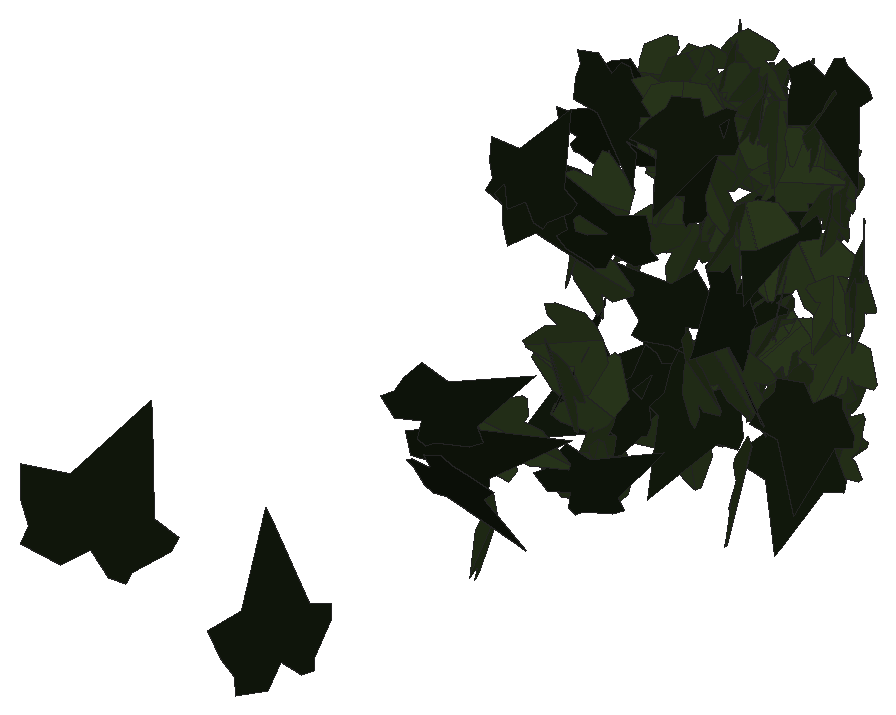
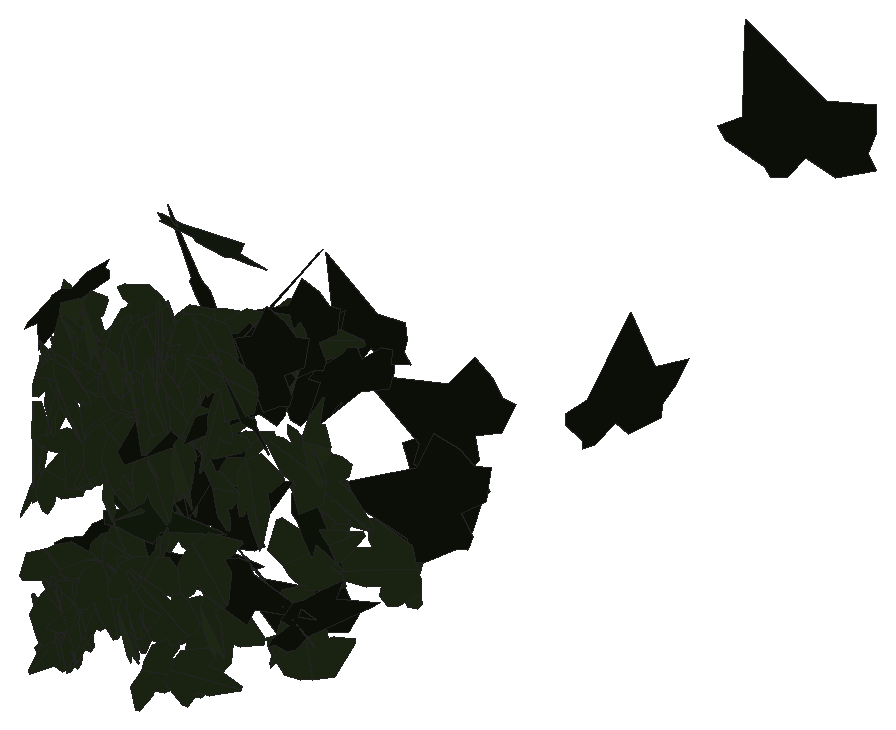
# SketchUp Ruby script. Lengths in inches.
U = 1.inch
M = Sketchup.active_model
def pt(a) = Geom::Point3d.new(a.map { |v| v * U })
def face(e, loops, mat)
  f = e.add_face(loops[0].map { |a| pt(a) })
  loops[1..].each { |l| e.add_face(l.map { |a| pt(a) }).erase! }
  f.material = f.back_material = mat if mat
  f
end
# faces: each face lists its corners as indices into pts; further lists are holes
def faces(e, pts, list, mat = nil) = list.each { |f| face(e, (f[0].is_a?(Array) ? f : [f]).map { |l| l.map { |i| pts[i] } }, mat) }
# xy, xz, yz: faces in a plane at the given z, y or x. An outline is a flat list of corners, or four numbers for a rectangle; further outlines are holes
def ring(l) = l.size == 4 ? [[l[0], l[1]], [l[2], l[1]], [l[2], l[3]], [l[0], l[3]]] : l.each_slice(2).to_a
def flat(e, list, mat, &to3) = list.each { |f| face(e, (f[0].is_a?(Array) ? f : [f]).map { |l| ring(l).map { |u, v| to3.(u, v) } }, mat) }
def xy(e, z, list, mat = nil) = flat(e, list, mat) { |x, y| [x, y, z] }
def xz(e, y, list, mat = nil) = flat(e, list, mat) { |x, z| [x, y, z] }
def yz(e, x, list, mat = nil) = flat(e, list, mat) { |y, z| [x, y, z] }
def lines(e, pts, list) = list.each { |a, b| e.add_line(pt(pts[a]), pt(pts[b])) }
# prism: a flat outline (further loops are holes) pulled along v
def prism(e, loops, v, mat = nil)
  f = face(e, loops, mat); d = Geom::Vector3d.new(v.map { |x| x * U })
  f.pushpull(f.normal.samedirection?(d) ? d.length : -d.length)
end
def box(e, o, s, mat = nil) = prism(e, [[o, [o[0] + s[0], o[1], o[2]], [o[0] + s[0], o[1] + s[1], o[2]], [o[0], o[1] + s[1], o[2]]]], [0, 0, s[2]], mat)
def at(x, y, z, deg = 0) = Geom::Transformation.translation(pt([x, y, z])) * Geom::Transformation.rotation(ORIGIN, Z_AXIS, deg.degrees)
def axes(o, x, y, z) = Geom::Transformation.new([*x, 0, *y, 0, *z, 0, *pt(o).to_a, 1])
def part(name) = M.definitions.add(name)
# library, detail: a bought-in or finely detailed component or shape, given as its bounding box
def library(name, o, s) = part(name).tap { |d| box(d.entities, o, s) }
def detail(e, o, s) = box(e.add_group.entities, o, s)
def put(e, d, t, mat = nil) = e.add_instance(d, t).tap { |i| i.material = mat if mat }
def group(e, t, mat = nil) = e.add_group.tap { |g| g.transformation = t; g.material = mat if mat }.entities
root = M.entities
M.materials.add("efeu1").color = [18, 25, 13]
M.materials.add("efeu2").color = [43, 57, 29]
c1 = part("ivyleaf_9")
p = [[1.54,2.16,1.25],[1.36,2.04,1.19],[-0.21,0.99,0.68],[-0.71,1.11,0.82],[-0.85,0.86,0.67],[-0.8,0.17,0.21],
  [-0.9,-0.01,0.1],[-0.67,-0.16,-0.02],[-0.08,-0.08,-0.05],[-0.03,-0.6,-0.4],[0.65,-0.88,-0.66],[0.83,-0.6,-0.49],
  [1.29,-0.42,-0.43],[1.8125,-0.07,-0.26],[1.21,0.44,0.15]]
faces(c1.entities,p,[[0,1,2,3,4,5,6,7,8,9,10,11,12,13,14]],"efeu1")
c2 = part("ivyleaf_10")
p = [[0,0.5,-0.03],[-0.0625,2.02,-0.43],[-0.19,2.01,-0.46],[-0.54,1.05,-0.29],[-0.52,0.625,-0.18],[-0.83,0.76,-0.28],
  [-1.16,0.64,-0.33],[-1.15,0.33,-0.24],[-0.77,-0.39,0.02],[-0.3,-0.51,0.16],[0.04,-0.48,0.23],[-0.02,2.01,-0.4375],
  [-0.06,2.01,-0.43],[0.04,-0.49,0.23],[0.67,-0.49,0.14],[1.38,0.36,-0.2],[1.375,0.51,-0.24],[0.81,0.65,-0.19],
  [0.62,0.59,-0.15],[0.6,1.09,-0.28],[0.5,1.23,-0.31]]
faces(c2.entities,p,[[0,1,2,3,4,5,6,7,8,9,10],[11,12,0,13,14,15,16,17,18,19,20]],"efeu2")
put(root,c1,axes([508.35,118,168.35],[-0.80992,-0.06692,0.86891],[0.90068,-0.17166,0.7642],[0.0905,1.10948,0.17065]))
put(root,c1,axes([509.34,122.875,163.92],[-0.48865,-0.70509,0.59701],[0.48935,0.38106,0.85817],[-0.85134,0.62373,0.1506]))
put(root,c1,axes([508.68,128.82,165.375],[0.90393,0.02313,0.05304],[0.05509,0.00026,-0.87078],[-0.02495,0.83852,-0.00119]))
put(root,c1,axes([508.39,128.84,166.52],[0.12124,-0.07324,0.85207],[0.88337,0.09754,-0.10749],[-0.09411,0.82118,0.08876]))
put(root,c2,axes([508.98,130.13,163.63],[0.02278,-0.05399,0.83347],[0.51986,-0.64094,-0.05808],[0.69446,0.48156,0.01614]))
put(root,c1,axes([508.17,129.62,165.1],[0.35904,0.07136,0.84573],[0.85849,0.17155,-0.35361],[-0.20067,0.86162,0.00036]))
put(root,c2,axes([507.93,131.74,164.78],[0.18066,0.06133,0.76871],[0.69913,0.35775,-0.18324],[-0.39096,0.66808,0.02755]))
put(root,c1,axes([508.29,132.27,170.14],[-0.51612,0.1888,0.56428],[0.50132,-0.28891,0.52976],[0.36555,0.66279,0.07018]))
put(root,c2,axes([508.98,132.43,166.39],[-0.65347,0.4003,-0.0382],[0.03066,-0.02366,-0.7545],[-0.43305,-0.60571,0.00423]))
put(root,c2,axes([509.32,132.85,166.89],[0.3552,-0.01331,-0.7252],[-0.73009,0.18356,-0.33524],[0.18529,0.74881,0.06929]))
put(root,c1,axes([509.14,132.74,163.37],[0.06641,-0.08518,0.72361],[0.75558,0.05107,-0.0578],[-0.04727,0.69662,0.09272]))
put(root,c2,axes([509.73,133.18,170.08],[0.14189,0.10505,0.76899],[-0.6514,-0.42782,0.17466],[0.47566,-0.61722,0.00981]))
put(root,c1,axes([508.04,132.89,170.07],[0.10578,-0.46737,-0.57412],[-0.04606,0.55237,-0.49423],[0.77981,0.09603,0.04869]))
put(root,c1,axes([509.67,133.29,168.9375],[0.44786,-0.10823,0.64797],[-0.64789,0.16839,0.44567],[-0.21608,-0.72924,0.00674]))
put(root,c2,axes([511.58,133.45,166.6875],[-0.04078,-0.01524,0.83192],[0.79397,-0.24982,0.03434],[0.24885,0.79457,0.02675]))
put(root,c2,axes([509.28,133.35,165.19],[0.39765,0.27834,0.62435],[-0.52526,-0.35203,0.47995],[0.4846,-0.60995,0.0079]))
put(root,c2,axes([508.94,133.43,163.01],[-0.62821,-0.33296,0.11741],[0.11317,0.04415,0.69689],[-0.36245,0.59088,0.01409]))
put(root,c1,axes([509.01,133.58,166.8],[-0.47671,0.28129,-0.44047],[0.36622,-0.25504,-0.5437],[-0.40915,-0.55602,0.02655]))
put(root,c1,axes([511.47,133.99,172.29],[-0.67868,-0.45976,-0.28208],[0.50624,-0.2748,-0.64498],[0.27585,-0.62685,0.48964]))
put(root,c2,axes([508.27,134.18,168.65],[0.18556,-0.29901,0.60908],[0.34703,-0.48995,-0.35818],[0.61961,0.36395,0.01821]))
put(root,c2,axes([509.19,133.26,164.01],[-0.00215,0.29168,0.64976],[-0.21374,0.59824,-0.29112],[-0.71332,-0.18014,0.08528]))
put(root,c2,axes([512.32,134.26,164.41],[0.34093,-0.41324,0.65956],[0.42905,-0.501,-0.53567],[0.64939,0.54796,0.00764]))
put(root,c2,axes([508.41,134.07,167.86],[0.00518,-0.01966,-0.8024],[0.7144,-0.39739,0.01481],[-0.42943,-0.66135,0.01495]))
put(root,c1,axes([511.13,133.92,170.55],[-0.23168,0.46867,0.64282],[0.27772,-0.57975,0.52278],[0.74548,0.36163,0.00502]))
put(root,c1,axes([508.42,133.89,170.88],[0.41242,-0.12481,0.56756],[0.55698,-0.17856,-0.41778],[0.23521,0.64169,-0.00586]))
put(root,c1,axes([508.36,134.66,164.6],[-0.35515,-0.43073,0.55439],[-0.32213,-0.45204,-0.55758],[0.62378,-0.47868,0.0277]))
put(root,c1,axes([508.78,134.43,172.15],[0.22842,-0.79499,0.10746],[0.0454,-0.09874,-0.827],[0.80094,0.23232,0.01623]))
put(root,c1,axes([511.7,134.77,167.94],[0.24173,-0.33736,-0.74303],[0.53299,-0.52154,0.41019],[-0.61792,-0.58183,0.06315]))
put(root,c1,axes([510.03,133.97,165.125],[-0.53393,0.49004,0.36474],[-0.27345,0.24144,-0.72469],[-0.54626,-0.59985,0.00627]))
put(root,c1,axes([510.9375,134.84,165.33],[-0.6752,-0.49233,-0.06076],[0.04867,0.03638,-0.83563],[0.49367,-0.67695,-0.00072]))
put(root,c1,axes([511.62,135.08,165.79],[0.17181,-0.35272,0.70217],[0.29434,-0.63754,-0.39228],[0.72858,0.34074,-0.00711]))
put(root,c2,axes([511.5,135.17,169.18],[-0.00977,0.06863,-0.73588],[0.02267,-0.73557,-0.0689],[-0.73873,-0.02348,0.00762]))
put(root,c2,axes([508.27,134.61,170.98],[-0.45655,0.59002,-0.14212],[0.07712,-0.11693,-0.75479],[-0.64953,-0.4286,0.01028]))
put(root,c2,axes([509.99,134.88,170.45],[0.67734,-0.34388,-0.02023],[-0.01714,0.01152,-0.74386],[0.37159,0.62736,0.00257]))
put(root,c2,axes([511.49,134.71,166.34],[-0.77683,0.00632,-0.33487],[0.33492,0.01008,-0.77676],[-0.00182,-0.84587,-0.01176]))
put(root,c1,axes([509.87,135.07,165.32],[-0.22912,-0.18393,-0.64949],[-0.54361,-0.37024,0.29123],[-0.44593,0.54584,-0.02132]))
put(root,c1,axes([510.06,135.12,166.57],[0.08917,-0.00641,0.70103],[-0.72077,0.09487,0.08595],[-0.10254,-0.67245,0.00544]))
put(root,c2,axes([508.96,134.93,171.56],[0.40955,0.49453,0.15605],[0.09784,0.11962,-0.64811],[-0.54949,0.38989,0.00091]))
put(root,c2,axes([510.25,135.03,164.26],[-0.66233,-0.4927,-0.06058],[0.04817,0.03673,-0.82549],[0.49407,-0.66408,-0.00072]))
put(root,c2,axes([510.58,135.2,170.14],[0.55853,-0.06915,0.5227],[0.54787,0.06062,-0.53419],[0.00753,0.7186,0.09536]))
put(root,c2,axes([511.61,135.47,169.33],[-0.72881,-0.23556,-0.29548],[0.39752,-0.38621,-0.5762],[0.02918,-0.62205,0.46963]))
put(root,c2,axes([509.49,135.64,168.47],[0.03444,0.17741,0.60964],[-0.1004,-0.57878,0.18744],[0.65378,-0.09822,-0.00333]))
put(root,c1,axes([513.06,135.61,165.42],[-0.22405,-0.73146,-0.03867],[0.01161,0.03689,-0.76501],[0.73239,-0.22435,0.00029]))
put(root,c1,axes([512.8125,135.66,164.3125],[-0.38444,-0.65055,-0.08061],[0.03708,0.07173,-0.75564],[0.65448,-0.3862,-0.00455]))
put(root,c2,axes([509.78,135.42,171.54],[0.70654,0.34748,0.00337],[0.00302,0.00164,-0.77039],[-0.37529,0.65421,0.00014]))
put(root,c2,axes([508.79,135.49,168.23],[0.09695,-0.71984,-0.06707],[-0.01625,0.06549,-0.7263],[0.72277,0.09803,-0.00733]))
put(root,c1,axes([511.91,136.09,169.36],[-0.60215,-0.49793,-0.32111],[0.58361,-0.27233,-0.55807],[0.24451,-0.57621,0.54124]))
put(root,c1,axes([507.98,135.58,171],[0.39146,-0.08579,0.64541],[0.63165,-0.13259,-0.40074],[0.15789,0.74311,0.00301]))
put(root,c2,axes([512.17,135.875,165.51],[-0.12287,-0.7097,-0.14698],[0.03958,0.14228,-0.72011],[0.72368,-0.12828,0.01443]))
put(root,c2,axes([510.89,136.42,168.84],[0.06532,-0.5106,0.52642],[0.10378,-0.51675,-0.5141],[0.72599,0.11981,0.02613]))
put(root,c1,axes([508.44,135.55,170.95],[0.58265,0.44586,0.21678],[0.16744,0.13789,-0.73363],[-0.46664,0.60619,0.00743]))
put(root,c2,axes([510.58,136.33,168.28],[0.18518,-0.45942,-0.41947],[0.22483,-0.34999,0.50664],[-0.6208,-0.26379,0.05836]))
put(root,c1,axes([511.39,136.38,166.97],[-0.69309,0.24528,-0.00723],[-0.18122,-0.45286,-0.50823],[-0.19336,-0.45476,0.50222]))
put(root,c2,axes([511.875,136.22,168.48],[0.07784,-0.63698,0.05729],[0.01392,-0.05602,-0.64168],[0.6394,0.07876,0.00699]))
put(root,c2,axes([509.89,136.4,168.78],[0.39324,-0.22962,0.57025],[0.5117,-0.2529,-0.4547],[0.34069,0.64488,0.02473]))
put(root,c1,axes([509.76,135.77,169.42],[0.23918,0.65563,-0.02342],[-0.01099,-0.02034,-0.7197],[-0.70841,0.22168,0.00325]))
put(root,c2,axes([509.66,136.08,170.94],[-0.65568,-0.31948,-0.21323],[0.19931,0.07762,-0.72917],[0.32834,-0.68509,0.01682]))
put(root,c2,axes([510.75,136.34,170.75],[-0.59006,-0.45413,0.18457],[-0.12783,-0.1363,-0.74402],[0.47325,-0.60305,0.02917]))
put(root,c2,axes([509.09,136.52,169.55],[0.16551,0.40545,0.51264],[-0.24613,-0.43875,0.44902],[0.64387,-0.27195,0.03987]))
put(root,c2,axes([509.13,136.52,171.45],[-0.17803,0.04055,-0.73109],[0.60563,-0.4147,-0.17048],[-0.41151,-0.62786,0.06538]))
put(root,c2,axes([511.92,136.32,170.02],[0.14883,-0.18809,-0.62528],[0.63899,-0.08999,0.17916],[-0.13434,-0.63642,0.15947]))
put(root,c2,axes([511.13,136.3125,171.5625],[0.18509,-0.59652,-0.18005],[-0.01518,0.18345,-0.6234],[0.62292,0.18172,0.03831]))
put(root,c2,axes([512.89,136.8125,167.43],[-0.17313,-0.38144,0.48849],[0.14492,-0.51805,-0.35316],[0.60259,0.015,0.22528]))
put(root,c2,axes([511.49,136.53,171.25],[0.01761,0.63966,-0.25407],[-0.00226,-0.2541,-0.63989],[-0.68827,0.0172,-0.0044]))
put(root,c2,axes([512.28,136.96,171.24],[-0.06052,-0.22027,-0.66498],[0.0953,-0.66384,0.21122],[-0.694,-0.07195,0.087]))
put(root,c1,axes([508.8,136.01,170.53],[-0.56172,0.25617,-0.54675],[-0.5119,0.19396,0.61679],[0.32019,0.7595,0.0269]))
put(root,c2,axes([512.14,136.64,168.18],[-0.69831,-0.24088,-0.42554],[0.5121,-0.29156,-0.60075],[0.02672,-0.70745,0.39248]))
put(root,c2,axes([509.33,136.41,171.875],[-0.45719,-0.34432,-0.23724],[0.19586,0.13853,-0.56746],[0.40077,-0.46049,0.00668]))
put(root,c2,axes([511.15,136.97,166.46],[0.0697,-0.43926,0.49745],[0.10397,-0.48679,-0.44441],[0.65544,0.12392,0.0176]))
put(root,c2,axes([512.68,136.96,169.6],[-0.06758,0.31516,-0.62508],[0.09975,-0.61725,-0.32199],[-0.6929,-0.11959,0.01461]))
put(root,c2,axes([508.88,136.8125,165.52],[0.27343,-0.45159,0.26163],[0.13523,-0.21821,-0.53842],[0.54167,0.28243,0.00235]))
put(root,c2,axes([511.52,136.93,169.79],[-0.24651,-0.50319,0.3595],[0.02692,-0.39538,-0.53494],[0.61783,-0.18355,0.16675]))
put(root,c2,axes([510.37,136.78,168.53],[-0.05221,-0.63909,0.12976],[-0.00411,-0.12985,-0.64119],[0.65212,-0.05199,0.00635]))
put(root,c2,axes([508.14,136.67,171.09],[0.10248,-0.06125,-0.70118],[0.68978,-0.13223,0.11236],[-0.14003,-0.69618,0.04035]))
put(root,c2,axes([510.24,136.76,166.54],[-0.08078,0.57633,-0.22736],[0.01515,-0.21857,-0.60425],[-0.66554,-0.07492,0.01384]))
put(root,c2,axes([509.71,136.95,170.48],[-0.25952,-0.53289,0.29073],[-0.0605,-0.2919,-0.58905],[0.60402,-0.2582,0.06591]))
put(root,c2,axes([511.76,136.9,165.31],[-0.066,0.58529,-0.36019],[0.04057,-0.3579,-0.589],[-0.68605,-0.07747,-0.00018]))
put(root,c2,axes([512.9,136.68,169.95],[-0.12207,-0.67095,-0.14265],[0.03341,0.1389,-0.68192],[0.68513,-0.12632,0.00783]))
put(root,c2,axes([510.39,136.93,171.68],[-0.30879,-0.54295,0.15479],[0.03751,-0.19577,-0.61186],[0.56334,-0.28458,0.12559]))
put(root,c2,axes([510.83,137.04,171.22],[0.00059,-0.57979,0.27924],[0.03094,-0.27889,-0.57913],[0.64279,0.01396,0.02762]))
put(root,c2,axes([509.48,136.94,169.08],[0.22232,-0.61813,0.11505],[0.05183,-0.1036,-0.65676],[0.62661,0.22788,0.01351]))
put(root,c2,axes([511.36,137.05,165.83],[-0.59465,0.23653,0.29391],[-0.39189,-0.43671,-0.35511],[0.06953,-0.43854,0.51216]))
put(root,c2,axes([510.58,137,171.65],[0.06509,-0.62126,0.15416],[0.05715,-0.1487,-0.62337],[0.63755,0.07676,0.04014]))
put(root,c2,axes([510.86,136.92,170.93],[-0.41578,0.25289,-0.44889],[0.38793,-0.22596,-0.4866],[-0.33907,-0.56861,-0.00627]))
put(root,c2,axes([511.21,136.64,170.25],[0.28524,0.60614,-0.14799],[0.02386,0.152,0.66858],[0.62349,-0.28312,0.04212]))
put(root,c2,axes([510.24,136.875,172.23],[-0.451,0.06488,-0.51754],[0.50231,-0.13028,-0.45406],[-0.14051,-0.674,0.03795]))
put(root,c2,axes([511.18,137.12,167.42],[0.42631,-0.41907,0.26503],[0.17459,-0.20028,-0.5975],[0.46409,0.4603,-0.01868]))
put(root,c2,axes([513.08,137.11,167.57],[-0.12451,0.50445,-0.38803],[0.0724,-0.38159,-0.51931],[-0.63229,-0.14303,0.01694]))
put(root,c1,axes([509.75,136.57,169.98],[0.02466,-0.13874,-0.68701],[0.05892,0.65919,-0.14202],[0.72662,-0.04874,0.03483]))
put(root,c2,axes([511.36,137.09,165.79],[-0.5098,-0.36935,-0.29326],[0.4735,-0.22076,-0.46254],[0.16633,-0.50358,0.41786]))
put(root,c1,axes([512.23,137.1,172.13],[0.17291,-0.73216,-0.23493],[-0.03547,0.23295,-0.75208],[0.76811,0.17557,0.01816]))
put(root,c2,axes([508.73,137.24,167.16],[-0.17583,-0.55983,0.28973],[-0.01528,-0.29692,-0.58299],[0.63017,-0.1634,0.0667]))
put(root,c2,axes([510.04,136.89,170.49],[-0.41989,-0.51086,-0.1733],[0.10947,0.13435,-0.66128],[0.52823,-0.43393,-0.00072]))
put(root,c2,axes([509.6875,137.17,171.06],[0.46251,-0.12014,0.4827],[0.46412,-0.13288,-0.47779],[0.17895,0.65517,-0.00839]))
put(root,c2,axes([512.4375,137.12,163.58],[0.46779,-0.20882,-0.40512],[0.36829,-0.16879,0.51227],[-0.26849,-0.59536,-0.00314]))
put(root,c2,axes([511.6,137.17,170.59],[-0.01252,-0.01891,0.72738],[0.72515,-0.0603,0.01092],[0.05998,0.72499,0.01988]))
put(root,c2,axes([508.66,136.84,168.59],[0.33387,-0.06081,0.61841],[-0.5927,0.17971,0.33766],[-0.18665,-0.67942,0.03396]))
put(root,c2,axes([512.66,136.62,163.94],[-0.06699,-0.29486,-0.60653],[0.14484,0.589,-0.30234],[0.65867,-0.15951,0.0048]))
put(root,c2,axes([510.42,137.2,165.14],[0.28586,-0.08671,0.58241],[0.57911,-0.07576,-0.29552],[0.10655,0.64434,0.04363]))
put(root,c2,axes([509.97,136.96,172.17],[0.21872,-0.58634,-0.24559],[0.02293,0.25413,-0.63733],[0.68229,0.17942,0.10015]))
put(root,c2,axes([509.84,137.47,164.25],[0.13708,0.32051,-0.57748],[-0.23829,-0.52606,-0.34854],[-0.61598,0.27483,0.00632]))
put(root,c2,axes([509.13,137.27,164.36],[0.16509,0.07816,-0.54894],[-0.53405,-0.18553,-0.17751],[-0.21651,0.51725,0.01928]))
put(root,c2,axes([510.9375,137.24,168.9],[-0.28687,-0.57109,0.16216],[-0.03787,-0.16213,-0.63798],[0.59246,-0.28689,0.03774]))
put(root,c2,axes([513.26,136.95,168.69],[0.24386,-0.55145,-0.29118],[-0.03765,0.29906,-0.59791],[0.62246,0.23413,0.07791]))
put(root,c2,axes([510.71,137.54,171.38],[0.16656,-0.4443,0.52296],[0.24083,-0.46607,-0.47267],[0.64257,0.28985,0.0416]))
put(root,c2,axes([512.1875,136.86,170.4],[0.35194,0.50858,-0.26519],[0.15546,0.2149,0.61845],[0.55209,-0.38471,-0.0051]))
put(root,c2,axes([512.55,137.25,165.81],[0.55429,0.251,-0.26853],[-0.2426,-0.11522,-0.60845],[-0.27615,0.60504,-0.00446]))
put(root,c2,axes([510.63,137.48,169.23],[-0.00418,-0.58535,0.3775],[0.04911,-0.37681,-0.58374],[0.69478,0.02311,0.04353]))
put(root,c2,axes([512.39,137.43,164.86],[-0.21486,-0.47748,0.38443],[-0.14978,-0.35412,-0.52355],[0.59443,-0.26182,0.00703]))
put(root,c2,axes([512.52,137.23,170.37],[0.66024,-0.31949,-0.08331],[-0.07484,0.03659,-0.73348],[0.32158,0.66447,0.00033]))
put(root,c2,axes([509.5625,137.04,165.23],[0.52803,0.05993,-0.48248],[0.48067,0.04268,0.53135],[0.07306,-0.71399,-0.00873]))
put(root,c2,axes([511.52,137.36,171.87],[0.26223,-0.57185,0.15686],[0.08817,-0.132,-0.62863],[0.58638,0.27558,0.02438]))
put(root,c2,axes([511.18,137.25,165.86],[-0.37357,-0.53152,0.10227],[-0.04541,-0.09305,-0.64947],[0.53936,-0.37597,0.01615]))
put(root,c2,axes([512.31,137.28,164.85],[0.37879,-0.5372,0.01208],[0.00355,-0.01227,-0.65731],[0.53733,0.37879,-0.00417]))
put(root,c2,axes([510.23,137.14,166.22],[-0.49556,-0.45076,-0.04619],[0.03426,0.03099,-0.6699],[0.45182,-0.49674,0.00013]))
put(root,c2,axes([511.16,136.84,169.03],[-0.21054,-0.39208,-0.52059],[0.24441,0.45965,-0.44503],[0.60415,-0.32258,-0.00138]))
put(root,c2,axes([509.875,137.3125,171.07],[0.11814,-0.62254,0.06343],[0.02136,-0.0605,-0.63358],[0.6254,0.11966,0.00966]))
put(root,c2,axes([512.24,137.32,164.95],[0.55797,-0.14282,0.29236],[0.29125,-0.03953,-0.57516],[0.14507,0.62868,0.03025]))
put(root,c2,axes([510.53,137.46,165.125],[0.28118,-0.46992,0.26744],[0.16265,-0.21018,-0.55801],[0.5552,0.29957,0.02803]))
put(root,c2,axes([512.4375,137.27,170.12],[0.6605,-0.26821,-0.18791],[-0.17482,0.06893,-0.71288],[0.27692,0.68324,-0.00184]))
put(root,c2,axes([511.76,137.01,164.75],[0.11642,0.70117,0.19962],[0.03318,0.19685,-0.71077],[-0.72828,0.12106,-0.00047]))
put(root,c2,axes([510.58,137.21,171.17],[0.24307,-0.60077,-0.15262],[-0.04763,0.14535,-0.648],[0.61802,0.24748,0.01009]))
put(root,c2,axes([508.51,136.92,170.57],[0.10833,-0.43705,-0.50066],[0.00704,0.48775,-0.45912],[0.70218,0.06253,0.08184]))
put(root,c2,axes([510.93,137.45,169.27],[-0.2568,-0.60586,0.22977],[-0.08116,-0.21514,-0.65798],[0.64286,-0.26918,0.00871]))
put(root,c2,axes([510.16,137.24,170.94],[-0.13904,-0.04039,0.69606],[0.68177,0.14078,0.14435],[-0.14603,0.69571,0.0112]))
